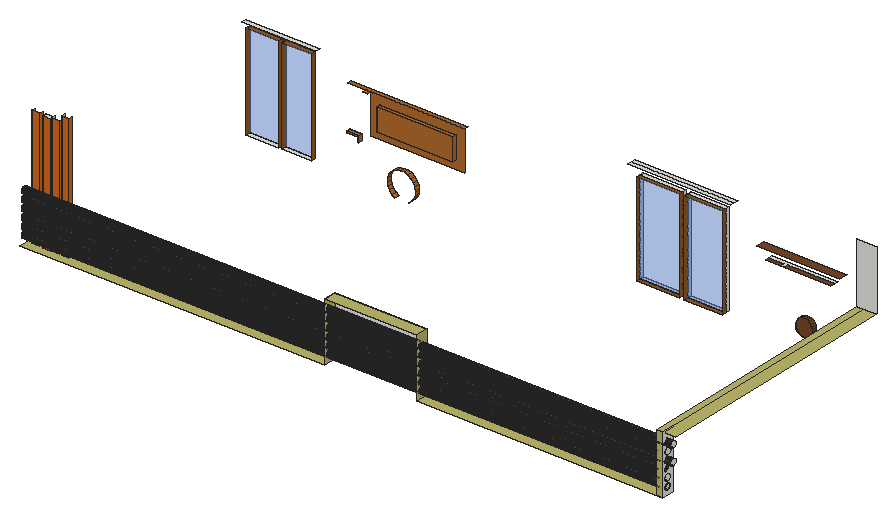
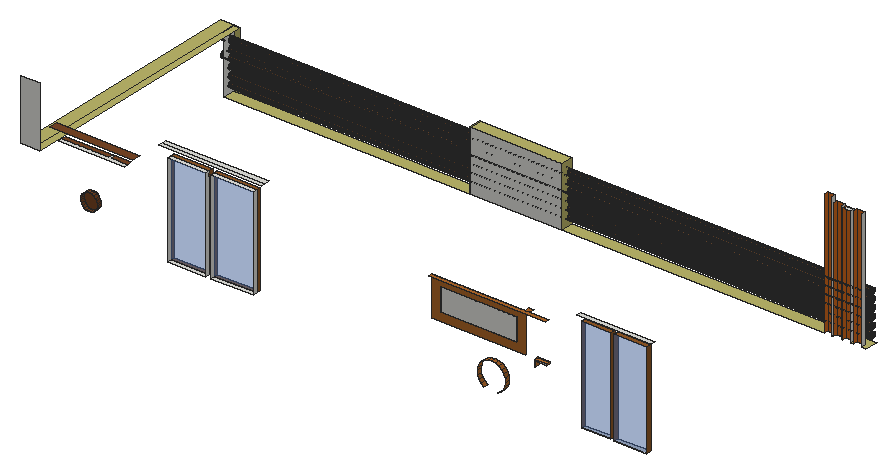
# SketchUp Ruby script. Lengths in inches.
U = 1.inch
M = Sketchup.active_model
def pt(a) = Geom::Point3d.new(a.map { |v| v * U })
def face(e, loops, mat)
  f = e.add_face(loops[0].map { |a| pt(a) })
  loops[1..].each { |l| e.add_face(l.map { |a| pt(a) }).erase! }
  f.material = f.back_material = mat if mat
  f
end
# faces: each face lists its corners as indices into pts; further lists are holes
def faces(e, pts, list, mat = nil) = list.each { |f| face(e, (f[0].is_a?(Array) ? f : [f]).map { |l| l.map { |i| pts[i] } }, mat) }
# xy, xz, yz: faces in a plane at the given z, y or x. An outline is a flat list of corners, or four numbers for a rectangle; further outlines are holes
def ring(l) = l.size == 4 ? [[l[0], l[1]], [l[2], l[1]], [l[2], l[3]], [l[0], l[3]]] : l.each_slice(2).to_a
def flat(e, list, mat, &to3) = list.each { |f| face(e, (f[0].is_a?(Array) ? f : [f]).map { |l| ring(l).map { |u, v| to3.(u, v) } }, mat) }
def xy(e, z, list, mat = nil) = flat(e, list, mat) { |x, y| [x, y, z] }
def xz(e, y, list, mat = nil) = flat(e, list, mat) { |x, z| [x, y, z] }
def yz(e, x, list, mat = nil) = flat(e, list, mat) { |y, z| [x, y, z] }
def lines(e, pts, list) = list.each { |a, b| e.add_line(pt(pts[a]), pt(pts[b])) }
# prism: a flat outline (further loops are holes) pulled along v
def prism(e, loops, v, mat = nil)
  f = face(e, loops, mat); d = Geom::Vector3d.new(v.map { |x| x * U })
  f.pushpull(f.normal.samedirection?(d) ? d.length : -d.length)
end
def box(e, o, s, mat = nil) = prism(e, [[o, [o[0] + s[0], o[1], o[2]], [o[0] + s[0], o[1] + s[1], o[2]], [o[0], o[1] + s[1], o[2]]]], [0, 0, s[2]], mat)
def at(x, y, z, deg = 0) = Geom::Transformation.translation(pt([x, y, z])) * Geom::Transformation.rotation(ORIGIN, Z_AXIS, deg.degrees)
def axes(o, x, y, z) = Geom::Transformation.new([*x, 0, *y, 0, *z, 0, *pt(o).to_a, 1])
def part(name) = M.definitions.add(name)
# library, detail: a bought-in or finely detailed component or shape, given as its bounding box
def library(name, o, s) = part(name).tap { |d| box(d.entities, o, s) }
def detail(e, o, s) = box(e.add_group.entities, o, s)
def put(e, d, t, mat = nil) = e.add_instance(d, t).tap { |i| i.material = mat if mat }
def group(e, t, mat = nil) = e.add_group.tap { |g| g.transformation = t; g.material = mat if mat }.entities
root = M.entities
M.materials.add("[0041_Chocolate]").color = [210, 105, 30]
M.materials.add("[0057_DarkKhaki]").color = [189, 183, 107]
M.materials.add("[Sandstone]").color = [118, 81, 52]
M.materials.add("[Translucent Glass Blue]").color = [100, 149, 237]
M.materials["[Translucent Glass Blue]"].alpha = 0.5
M.materials.add("[Wood Bamboo]").color = [177, 105, 43]
M.materials.add("[Wood Floor Parquet]").color = [145, 89, 39]
M.materials.add("[Wood Veneer 01]").color = [120, 70, 37]
xy(root,144,[[9,12,227.54,12,227.54,21,39.11,21,39.11,18.25,33.61,18.25,33.61,21,32.36,21,32.36,18.25,26.86,18.25,26.86,21,25.61,21,25.61,18.25,20.11,18.25,20.11,21,17.86,21,17.86,18.25,12.36,18.25,12.36,21,9,21],[293.97,12,471,21]],"[0057_DarkKhaki]")
xy(root,144.78,[[29.52,189.3,53.11,192.3],[55.4,189.3,76.7,192.3]])
xy(root,149.36,[[310,192.3,340.91,195.3],[344.375,192.3,371.82,195.3]])
xy(root,149.36,[[310,189.3,340.91,192.3],[344.375,189.3,371.82,192.3]],"[Wood Floor Parquet]")
xy(root,170.25,[[112.03,186.3,112.78,189.3]])
xy(root,173.75,[[104.03,186.3,112.03,189.3]],"[Wood Bamboo]")
xy(root,174.75,[[104.03,186.3,112.78,189.3]],"[Wood Bamboo]")
xy(root,181.75,[[125.53,186.3,180.32,189.3]],"[Wood Bamboo]")
xy(root,186.25,[[466.21,12,471,192.3],[471,12,480,192.3]],"[0057_DarkKhaki]")
xy(root,186.625,[[227.54,12,293.97,21]],"[0057_DarkKhaki]")
xy(root,197.62,[[416.3125,186.3,416.3125,189.3,405.17,189.3,405.17,192.3,452.41,192.3,452.41,189.3,418.65,189.3,418.65,186.3]])
xy(root,197.62,[[405.17,186.3,416.3125,189.3],[418.65,186.3,452.41,189.3]],"[Wood Veneer 01]")
xy(root,197.82,[[125.53,186.3,180.32,189.3]],"[Wood Bamboo]")
xy(root,204,[[115.97,186.3,119.35,189.3],[102.5,189.3,186.5,192.3]],"[Wood Bamboo]")
xy(root,204,[[398.79,186.3,458.79,192.3]],"[Wood Veneer 01]")
xy(root,213.4,[[29.52,189.3,53.11,192.3],[55.4,189.3,76.7,192.3]],"[Wood Floor Parquet]")
xy(root,216.18,[[310,192.3,340.91,195.3],[344.375,192.3,371.82,195.3]])
xy(root,216.18,[[310,189.3,340.91,192.3],[344.375,189.3,371.82,192.3]],"[Wood Floor Parquet]")
xy(root,216.4,[[26.52,189.3,79.7,192.3]])
xy(root,222.24,[[303.94,189.3,377.89,192.3],[303.94,192.3,377.89,195.3]])
xy(root,229,[[20.11,18.25,25.61,21]])
xz(root,12,[[466.21,144,471,186.25]],"[0057_DarkKhaki]")
xz(root,18.25,[[12.36,144,17.86,229.6875],[20.11,144,25.61,229],[26.86,144,32.36,229.6875],[33.61,144,39.11,233.5625]],"[0041_Chocolate]")
xz(root,21,[[227.54,144,293.97,186.625]])
xz(root,186.3,[[112.03,170.25,112.78,170.25,112.78,174.75,104.03,174.75,104.03,173.75,112.03,173.75],[125.53,181.75,180.32,197.82]],"[Wood Bamboo]")
xz(root,186.3,[[433.6,157.54,435.15,157.92,436.56,158.68,437.71,159.79,438.54,161.15,438.99,162.6875,439.03,164.29,438.65,165.84,437.88,167.24,436.78,168.4,435.41,169.23,433.88,169.68,432.28,169.72,430.73,169.34,429.32,168.57,428.17,167.47,427.34,166.1,426.89,164.57,426.85,162.97,427.23,161.41,428,160.01,429.1,158.85,430.47,158.02,432,157.57]],"[Wood Veneer 01]")
xz(root,189.3,[[112.03,170.25,112.03,173.75,104.03,173.75,104.03,174.75,112.78,174.75,112.78,170.25],[125.53,181.75,180.32,197.82]])
xz(root,189.3,[[[119.35,175.57,186.5,204],[125.53,181.75,180.32,197.82]]],"[Wood Bamboo]")
xz(root,192.3,[[466.21,186.25,480,229.6875]])
xz(root,192.3,[[29.52,144.78,53.11,213.4],[55.4,144.78,76.7,213.4],[310,149.36,340.91,216.18],[344.375,149.36,371.82,216.18]],"[Translucent Glass Blue]")
yz(root,12.36,[[18.25,144,21,229.6875]])
yz(root,17.86,[[18.25,144,21,229.6875]],"[0041_Chocolate]")
yz(root,20.11,[[18.25,144,21,229]])
yz(root,25.61,[[18.25,144,21,229]],"[0041_Chocolate]")
yz(root,26.86,[[18.25,144,21,229.6875]])
yz(root,29.52,[[189.3,144.78,192.3,213.4]],"[Wood Floor Parquet]")
yz(root,32.36,[[18.25,144,21,229.6875]],"[0041_Chocolate]")
yz(root,33.61,[[18.25,144,21,233.5625]])
yz(root,39.11,[[18.25,144,21,233.5625]],"[0041_Chocolate]")
yz(root,53.11,[[189.3,144.78,192.3,213.4]],"[Wood Floor Parquet]")
yz(root,55.4,[[189.3,144.78,192.3,213.4]],"[Wood Floor Parquet]")
yz(root,76.7,[[189.3,144.78,192.3,213.4]],"[Wood Floor Parquet]")
yz(root,104.03,[[186.3,173.75,189.3,174.75]],"[Wood Bamboo]")
yz(root,112.03,[[186.3,170.25,189.3,173.75]],"[Wood Bamboo]")
yz(root,112.78,[[186.3,170.25,189.3,174.75]],"[Wood Bamboo]")
yz(root,125.53,[[186.3,181.75,189.3,197.82]],"[Wood Bamboo]")
yz(root,180.32,[[186.3,181.75,189.3,197.82]],"[Wood Bamboo]")
yz(root,227.54,[[12,144,21,186.625]],"[0057_DarkKhaki]")
yz(root,293.97,[[12,144,21,186.625]],"[0057_DarkKhaki]")
yz(root,310,[[192.3,149.36,195.3,216.18]])
yz(root,310,[[189.3,149.36,192.3,216.18]],"[Wood Floor Parquet]")
yz(root,340.91,[[192.3,149.36,195.3,216.18]])
yz(root,340.91,[[189.3,149.36,192.3,216.18]],"[Wood Floor Parquet]")
yz(root,344.375,[[192.3,149.36,195.3,216.18]])
yz(root,344.375,[[189.3,149.36,192.3,216.18]],"[Wood Floor Parquet]")
yz(root,371.82,[[192.3,149.36,195.3,216.18]])
yz(root,371.82,[[189.3,149.36,192.3,216.18]],"[Wood Floor Parquet]")
yz(root,471,[[[12,144,21,186.25],[15.06,159.57,15.61,159.65,16.12,159.86,16.56,160.2,16.9,160.64,17.11,161.15,17.18,161.7,17.11,162.25,16.9,162.76,16.56,163.2,16.12,163.54,15.61,163.75,15.06,163.82,14.51,163.75,13.99,163.54,13.55,163.2,13.21,162.76,13,162.25,12.93,161.7,13,161.15,13.21,160.64,13.55,160.2,13.99,159.86,14.51,159.65]]])
yz(root,471.8125,[[15.06,153.89,15.61,153.96,16.12,154.17,16.56,154.51,16.9,154.95,17.11,155.46,17.18,156.01,17.11,156.5625,16.9,157.07,16.56,157.51,16.12,157.85,15.61,158.0625,15.06,158.14,14.51,158.0625,13.99,157.85,13.55,157.51,13.21,157.07,13,156.5625,12.93,156.01,13,155.46,13.21,154.95,13.55,154.51,13.99,154.17,14.51,153.96]])
yz(root,472.125,[[15.06,170.95,15.61,171.02,16.12,171.23,16.56,171.57,16.9,172.01,17.11,172.52,17.18,173.07,17.11,173.625,16.9,174.14,16.56,174.58,16.12,174.91,15.61,175.125,15.06,175.2,14.51,175.125,13.99,174.91,13.55,174.58,13.21,174.14,13,173.625,12.93,173.07,13,172.52,13.21,172.01,13.55,171.57,13.99,171.23,14.51,171.02]])
yz(root,476.0625,[[15.06,165.26,15.61,165.33,16.12,165.55,16.56,165.88,16.9,166.32,17.11,166.84,17.18,167.39,17.11,167.9375,16.9,168.45,16.56,168.89,16.12,169.23,15.61,169.4375,15.06,169.51,14.51,169.4375,13.99,169.23,13.55,168.89,13.21,168.45,13,167.9375,12.93,167.39,13,166.84,13.21,166.32,13.55,165.88,13.99,165.55,14.51,165.33]])
yz(root,476.125,[[15.06,176.64,15.61,176.71,16.12,176.92,16.56,177.26,16.9,177.7,17.11,178.21,17.18,178.76,17.11,179.3125,16.9,179.82,16.56,180.26,16.12,180.6,15.61,180.8125,15.06,180.89,14.51,180.8125,13.99,180.6,13.55,180.26,13.21,179.82,13,179.3125,12.93,178.76,13,178.21,13.21,177.7,13.55,177.26,13.99,176.92,14.51,176.71]])
p = [[136.75,189.3,145.44],[138.92,189.3,143.91],[138.92,186.3,143.91],[136.75,186.3,145.44],[149.1,189.3,144.31],[151.14,189.3,146.01],
  [151.14,186.3,146.01],[149.1,186.3,144.31],[135.05,189.3,147.49],[135.05,186.3,147.49],[152.68,189.3,148.18],[152.68,186.3,148.18],
  [133.93,189.3,149.9],[133.93,186.3,149.9],[9,13.99,148.36],[9,14.51,148.15],[471.8125,14.51,148.15],[471.8125,13.99,148.36],
  [9,15.06,148.07],[471.8125,15.06,148.07],[9,15.61,148.15],[471.8125,15.61,148.15],[9,16.12,148.36],[471.8125,16.12,148.36],
  [153.6,189.3,150.67],[153.6,186.3,150.67],[9,13.55,148.7],[471.8125,13.55,148.7],[9,16.56,148.7],[471.8125,16.56,148.7],
  [9,13.21,149.14],[471.8125,13.21,149.14],[9,16.9,149.14],[471.8125,16.9,149.14],[9,13,149.65],[471.8125,13,149.65],
  [9,17.11,149.65],[471.8125,17.11,149.65],[9,12.93,150.2],[471.8125,12.93,150.2],[9,17.18,150.2],[471.8125,17.18,150.2],
  [133.48,189.3,152.52],[133.48,186.3,152.52],[9,13,150.75],[471.8125,13,150.75],[9,17.11,150.75],[471.8125,17.11,150.75],
  [9,13.21,151.26],[471.8125,13.21,151.26],[9,16.9,151.26],[471.8125,16.9,151.26],[153.84,189.3,153.32],[153.84,186.3,153.32],
  [9,13.55,151.7],[471.8125,13.55,151.7],[9,16.56,151.7],[471.8125,16.56,151.7],[9,13.99,152.04],[471.8125,13.99,152.04],
  [9,16.12,152.04],[471.8125,16.12,152.04],[9,14.51,152.25],[471.8125,14.51,152.25],[9,15.61,152.25],[471.8125,15.61,152.25],
  [9,15.06,152.32],[471.8125,15.06,152.32],[133.73,189.3,155.17],[133.73,186.3,155.17],[153.39,189.3,155.94],[153.39,186.3,155.94],
  [9,14.51,153.96],[9,15.06,153.89],[471.8125,15.06,153.89],[471.8125,14.51,153.96],[9,15.61,153.96],[471.8125,15.61,153.96],
  [9,13.99,154.17],[471.8125,13.99,154.17],[9,16.12,154.17],[471.8125,16.12,154.17],[9,13.55,154.51],[471.8125,13.55,154.51],
  [9,16.56,154.51],[471.8125,16.56,154.51],[9,13.21,154.95],[471.8125,13.21,154.95],[9,16.9,154.95],[471.8125,16.9,154.95],
  [9,13,155.46],[471.8125,13,155.46],[9,17.11,155.46],[471.8125,17.11,155.46],[134.65,189.3,157.67],[134.65,186.3,157.67],
  [9,12.93,156.01],[471.8125,12.93,156.01],[9,17.18,156.01],[471.8125,17.18,156.01],[152.28,189.3,158.36],[152.28,186.3,158.36],
  [9,13,156.5625],[471.8125,13,156.5625],[9,17.11,156.5625],[471.8125,17.11,156.5625],[9,13.21,157.07],[471.8125,13.21,157.07],
  [9,16.9,157.07],[471.8125,16.9,157.07],[9,13.55,157.51],[471.8125,13.55,157.51],[9,16.56,157.51],[471.8125,16.56,157.51],
  [9,13.99,157.85],[471.8125,13.99,157.85],[9,16.12,157.85],[471.8125,16.12,157.85],[432,189.3,157.57],[433.6,189.3,157.54],
  [433.6,186.3,157.54],[432,186.3,157.57],[435.15,189.3,157.92],[435.15,186.3,157.92],[430.47,189.3,158.02],[430.47,186.3,158.02],
  [136.18,189.3,159.84],[136.18,186.3,159.84],[9,14.51,158.0625],[471.8125,14.51,158.0625],[9,15.61,158.0625],[471.8125,15.61,158.0625],
  [436.56,189.3,158.68],[436.56,186.3,158.68],[429.1,189.3,158.85],[429.1,186.3,158.85],[9,15.06,158.14],[471.8125,15.06,158.14],
  [150.58,189.3,160.4],[150.58,186.3,160.4],[437.71,189.3,159.79],[437.71,186.3,159.79],[428,189.3,160.01],[428,186.3,160.01],
  [9,13.99,159.86],[9,14.51,159.65],[471,14.51,159.65],[471,13.99,159.86],[9,15.06,159.57],[471,15.06,159.57],
  [9,15.61,159.65],[471,15.61,159.65],[9,16.12,159.86],[471,16.12,159.86],[138.23,189.3,161.54],[138.23,186.3,161.54],
  [438.54,189.3,161.15],[438.54,186.3,161.15],[9,13.55,160.2],[471,13.55,160.2],[9,16.56,160.2],[471,16.56,160.2],
  [427.23,189.3,161.41],[427.23,186.3,161.41],[9,13.21,160.64],[471,13.21,160.64],[9,16.9,160.64],[471,16.9,160.64],
  [148.41,189.3,161.9375],[148.41,186.3,161.9375],[9,13,161.15],[471,13,161.15],[9,17.11,161.15],[471,17.11,161.15],
  [9,12.93,161.7],[471,12.93,161.7],[9,17.18,161.7],[471,17.18,161.7],[438.99,189.3,162.6875],[438.99,186.3,162.6875],
  [426.85,189.3,162.97],[426.85,186.3,162.97],[140.64,189.3,162.65],[140.64,186.3,162.65],[9,13,162.25],[471,13,162.25],
  [9,17.11,162.25],[471,17.11,162.25],[145.91,189.3,162.86],[145.91,186.3,162.86],[9,13.21,162.76],[471,13.21,162.76],
  [9,16.9,162.76],[471,16.9,162.76],[143.26,189.3,163.1],[143.26,186.3,163.1],[439.03,189.3,164.29],[439.03,186.3,164.29],
  [9,13.55,163.2],[471,13.55,163.2],[9,16.56,163.2],[471,16.56,163.2],[426.89,189.3,164.57],[426.89,186.3,164.57],
  [9,13.99,163.54],[471,13.99,163.54],[9,16.12,163.54],[471,16.12,163.54],[9,14.51,163.75],[471,14.51,163.75],
  [9,15.61,163.75],[471,15.61,163.75],[9,15.06,163.82],[471,15.06,163.82],[438.65,189.3,165.84],[438.65,186.3,165.84],
  [427.34,189.3,166.1],[427.34,186.3,166.1],[9,13.99,165.55],[9,14.51,165.33],[476.0625,14.51,165.33],[476.0625,13.99,165.55],
  [9,15.06,165.26],[476.0625,15.06,165.26],[9,15.61,165.33],[476.0625,15.61,165.33],[9,16.12,165.55],[476.0625,16.12,165.55],
  [9,13.55,165.88],[476.0625,13.55,165.88],[9,16.56,165.88],[476.0625,16.56,165.88],[437.88,189.3,167.24],[437.88,186.3,167.24],
  [9,13.21,166.32],[476.0625,13.21,166.32],[9,16.9,166.32],[476.0625,16.9,166.32],[428.17,189.3,167.47],[428.17,186.3,167.47],
  [9,13,166.84],[476.0625,13,166.84],[9,17.11,166.84],[476.0625,17.11,166.84],[9,12.93,167.39],[476.0625,12.93,167.39],
  [9,17.18,167.39],[476.0625,17.18,167.39],[436.78,189.3,168.4],[436.78,186.3,168.4],[9,13,167.9375],[476.0625,13,167.9375],
  [9,17.11,167.9375],[476.0625,17.11,167.9375],[429.32,189.3,168.57],[429.32,186.3,168.57],[9,13.21,168.45],[476.0625,13.21,168.45],
  [9,16.9,168.45],[476.0625,16.9,168.45],[9,13.55,168.89],[476.0625,13.55,168.89],[9,16.56,168.89],[476.0625,16.56,168.89],
  [435.41,189.3,169.23],[435.41,186.3,169.23],[430.73,189.3,169.34],[430.73,186.3,169.34],[9,13.99,169.23],[476.0625,13.99,169.23],
  [9,16.12,169.23],[476.0625,16.12,169.23],[9,14.51,169.4375],[476.0625,14.51,169.4375],[9,15.61,169.4375],[476.0625,15.61,169.4375],
  [433.88,189.3,169.68],[433.88,186.3,169.68],[432.28,189.3,169.72],[432.28,186.3,169.72],[9,15.06,169.51],[476.0625,15.06,169.51],
  [9,14.51,171.02],[9,15.06,170.95],[472.125,15.06,170.95],[472.125,14.51,171.02],[9,15.61,171.02],[472.125,15.61,171.02],
  [9,13.99,171.23],[472.125,13.99,171.23],[9,16.12,171.23],[472.125,16.12,171.23],[9,13.55,171.57],[472.125,13.55,171.57],
  [9,16.56,171.57],[472.125,16.56,171.57],[9,13.21,172.01],[472.125,13.21,172.01],[9,16.9,172.01],[472.125,16.9,172.01],
  [9,13,172.52],[472.125,13,172.52],[9,17.11,172.52],[472.125,17.11,172.52],[9,12.93,173.07],[472.125,12.93,173.07],
  [9,17.18,173.07],[472.125,17.18,173.07],[9,13,173.625],[472.125,13,173.625],[9,17.11,173.625],[472.125,17.11,173.625],
  [9,13.21,174.14],[472.125,13.21,174.14],[9,16.9,174.14],[472.125,16.9,174.14],[9,13.55,174.58],[472.125,13.55,174.58],
  [9,16.56,174.58],[472.125,16.56,174.58],[9,13.99,174.91],[472.125,13.99,174.91],[9,16.12,174.91],[472.125,16.12,174.91],
  [9,14.51,175.125],[472.125,14.51,175.125],[9,15.61,175.125],[472.125,15.61,175.125],[9,15.06,175.2],[472.125,15.06,175.2],
  [9,14.51,176.71],[9,15.06,176.64],[476.125,15.06,176.64],[476.125,14.51,176.71],[9,15.61,176.71],[476.125,15.61,176.71],
  [9,13.99,176.92],[476.125,13.99,176.92],[9,16.12,176.92],[476.125,16.12,176.92],[9,13.55,177.26],[476.125,13.55,177.26],
  [9,16.56,177.26],[476.125,16.56,177.26],[9,13.21,177.7],[476.125,13.21,177.7],[9,16.9,177.7],[476.125,16.9,177.7],
  [9,13,178.21],[476.125,13,178.21],[9,17.11,178.21],[476.125,17.11,178.21],[9,12.93,178.76],[476.125,12.93,178.76],
  [9,17.18,178.76],[476.125,17.18,178.76],[9,13,179.3125],[476.125,13,179.3125],[9,17.11,179.3125],[476.125,17.11,179.3125],
  [9,13.21,179.82],[476.125,13.21,179.82],[9,16.9,179.82],[476.125,16.9,179.82],[9,13.55,180.26],[476.125,13.55,180.26],
  [9,16.56,180.26],[476.125,16.56,180.26],[9,13.99,180.6],[476.125,13.99,180.6],[9,16.12,180.6],[476.125,16.12,180.6],
  [9,14.51,180.8125],[476.125,14.51,180.8125],[9,15.61,180.8125],[476.125,15.61,180.8125],[9,15.06,180.89],[476.125,15.06,180.89]]
faces(root,p,[[0,1,2,3],[4,5,6,7],[8,0,3,9],[5,10,11,6],[12,8,9,13],[10,24,25,11],[42,12,13,43],[24,52,53,25],
  [68,42,43,69],[52,70,71,53],[94,68,69,95],[70,100,101,71],[126,94,95,127],[100,138,139,101],[154,126,127,155],[138,168,169,139],
  [182,154,155,183],[168,188,189,169],[194,182,183,195],[188,194,195,189]],"[Wood Bamboo]")
faces(root,p,[[14,15,16,17],[15,18,19,16],[18,20,21,19],[20,22,23,21],[26,14,17,27],[22,28,29,23],[30,26,27,31],[28,32,33,29],
  [34,30,31,35],[32,36,37,33],[38,34,35,39],[36,40,41,37],[44,38,39,45],[40,46,47,41],[48,44,45,49],[46,50,51,47],
  [54,48,49,55],[50,56,57,51],[58,54,55,59],[56,60,61,57],[62,58,59,63],[60,64,65,61],[66,62,63,67],[64,66,67,65],
  [72,73,74,75],[73,76,77,74],[78,72,75,79],[76,80,81,77],[82,78,79,83],[80,84,85,81],[86,82,83,87],[84,88,89,85],
  [90,86,87,91],[88,92,93,89],[96,90,91,97],[92,98,99,93],[102,96,97,103],[98,104,105,99],[106,102,103,107],[104,108,109,105],
  [110,106,107,111],[108,112,113,109],[114,110,111,115],[112,116,117,113],[128,114,115,129],[116,130,131,117],[136,128,129,137],[130,136,137,131],
  [144,145,146,147],[145,148,149,146],[148,150,151,149],[150,152,153,151],[158,144,147,159],[152,160,161,153],[164,158,159,165],[160,166,167,161],
  [170,164,165,171],[166,172,173,167],[174,170,171,175],[172,176,177,173],[184,174,175,185],[176,186,187,177],[190,184,185,191],[186,192,193,187],
  [198,190,191,199],[192,200,201,193],[204,198,199,205],[200,206,207,201],[208,204,205,209],[206,210,211,207],[212,208,209,213],[210,212,213,211],
  [218,219,220,221],[219,222,223,220],[222,224,225,223],[224,226,227,225],[228,218,221,229],[226,230,231,227],[234,228,229,235],[230,236,237,231],
  [240,234,235,241],[236,242,243,237],[244,240,241,245],[242,246,247,243],[250,244,245,251],[246,252,253,247],[256,250,251,257],[252,258,259,253],
  [260,256,257,261],[258,262,263,259],[268,260,261,269],[262,270,271,263],[272,268,269,273],[270,274,275,271],[280,272,273,281],[274,280,281,275],
  [282,283,284,285],[283,286,287,284],[288,282,285,289],[286,290,291,287],[292,288,289,293],[290,294,295,291],[296,292,293,297],[294,298,299,295],
  [300,296,297,301],[298,302,303,299],[304,300,301,305],[302,306,307,303],[308,304,305,309],[306,310,311,307],[312,308,309,313],[310,314,315,311],
  [316,312,313,317],[314,318,319,315],[320,316,317,321],[318,322,323,319],[324,320,321,325],[322,326,327,323],[328,324,325,329],[326,328,329,327],
  [330,331,332,333],[331,334,335,332],[336,330,333,337],[334,338,339,335],[340,336,337,341],[338,342,343,339],[344,340,341,345],[342,346,347,343],
  [348,344,345,349],[346,350,351,347],[352,348,349,353],[350,354,355,351],[356,352,353,357],[354,358,359,355],[360,356,357,361],[358,362,363,359],
  [364,360,361,365],[362,366,367,363],[368,364,365,369],[366,370,371,367],[372,368,369,373],[370,374,375,371],[376,372,373,377],[374,376,377,375]],"[Sandstone]")
faces(root,p,[[118,119,120,121],[119,122,123,120],[124,118,121,125],[122,132,133,123],[134,124,125,135],[132,140,141,133],[142,134,135,143],[140,156,157,141],
  [162,142,143,163],[156,178,179,157],[180,162,163,181],[178,196,197,179],[202,180,181,203],[196,214,215,197],[216,202,203,217],[214,232,233,215],
  [238,216,217,239],[232,248,249,233],[254,238,239,255],[248,264,265,249],[266,254,255,267],[264,276,277,265],[278,266,267,279],[276,278,279,277]],"[Wood Veneer 01]")
